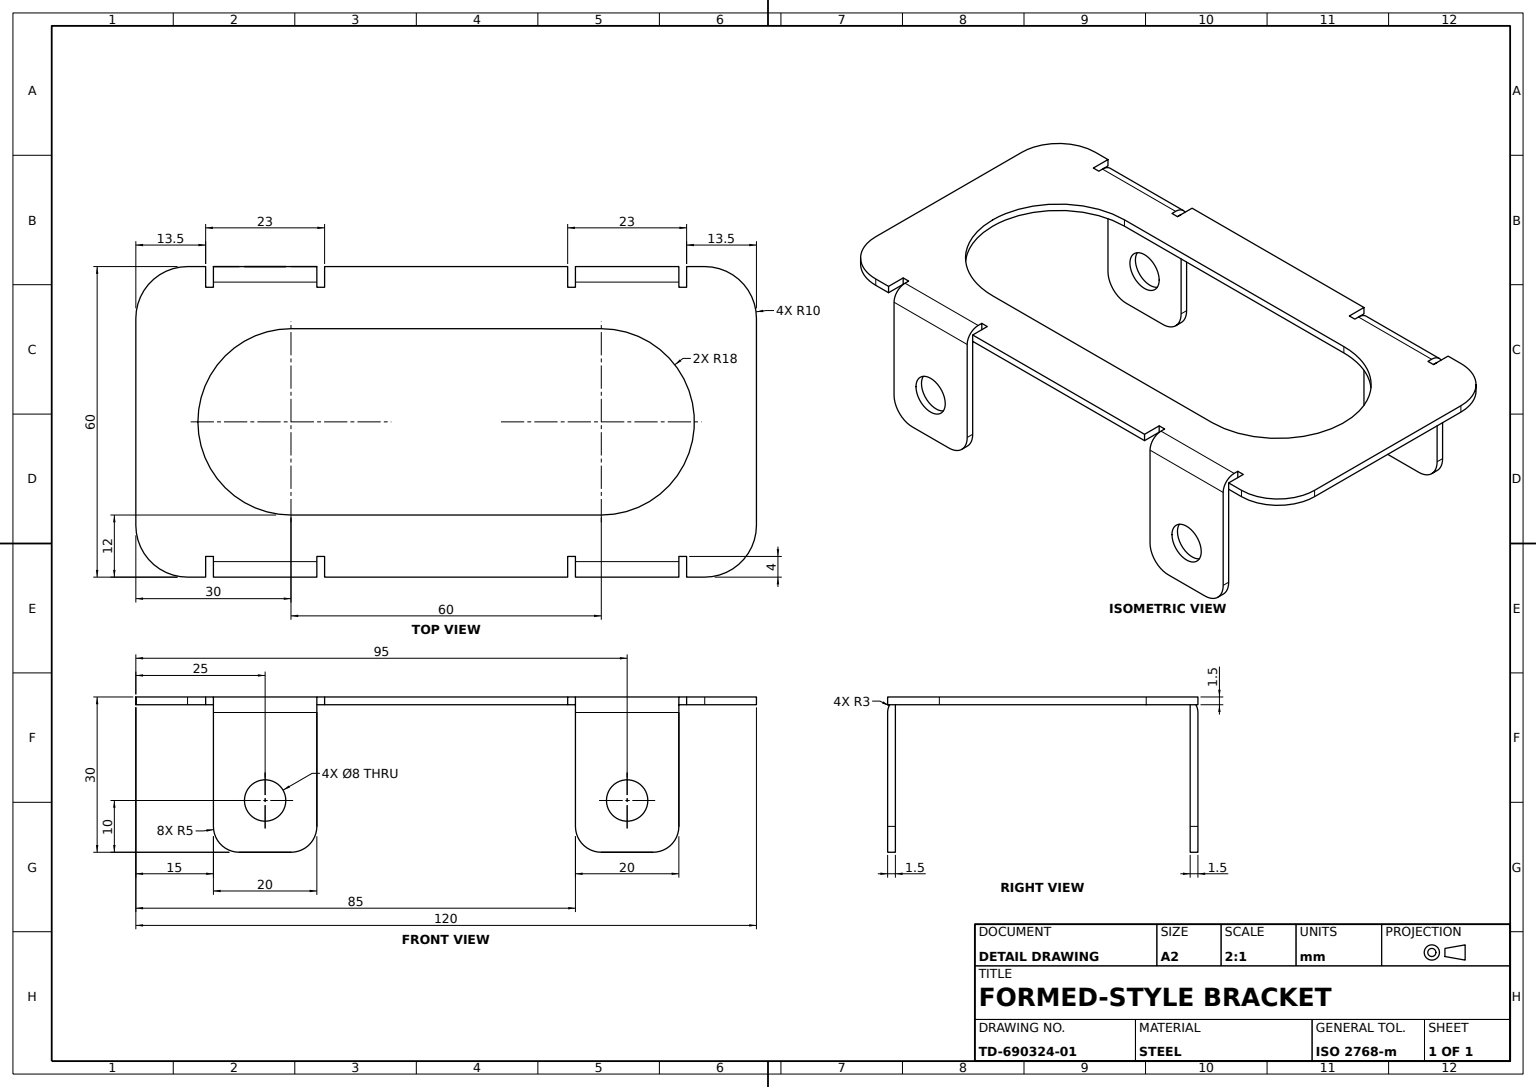
solid
v1 (-28.5,-18.5,39)
v2 (-28.5,-18.5,31)
e1 v1 v2 CIRCLE(AX(P(-28.5,-18.5,35),D(-1,0,0),D(0,0,1)),4)
e2 v2 v1 CIRCLE(AX(P(-28.5,-18.5,35),D(-1,0,0),D(0,0,1)),4)
v3 (-28.5,0,25)
v4 (-28.5,0,45)
e3 v3 v4 LINE
v5 (-28.5,-23.5,45)
e4 v5 v4 LINE
v6 (-28.5,-28.5,40)
e5 v6 v5 CIRCLE(AX(P(-28.5,-23.5,40),D(-1,0,0),D(0,0,1)),5)
v7 (-28.5,-28.5,30)
e6 v7 v6 LINE
v8 (-28.5,-23.5,25)
e7 v8 v7 CIRCLE(AX(P(-28.5,-23.5,30),D(-1,0,0),D(0,0,1)),5)
e8 v3 v8 LINE
face PLANE(AX(P(-28.5,-23.5,30),D(-1,0,0),D(0,0,1))) rev [e1 e2] [e3 -e4 -e5 -e6 -e7 -e8]
v9 (-30,-18.5,-39)
v10 (-30,-18.5,-31)
e9 v9 v10 CIRCLE(AX(P(-30,-18.5,-35),D(-1,0,0),D(0,0,1)),4)
e10 v10 v9 CIRCLE(AX(P(-30,-18.5,-35),D(-1,0,0),D(0,0,1)),4)
v11 (-30,-28.5,-40)
v12 (-30,-28.5,-30)
e11 v11 v12 LINE
v13 (-30,-23.5,-25)
e12 v12 v13 CIRCLE(AX(P(-30,-23.5,-30),D(-1,0,0),D(0,0,1)),5)
v14 (-30,-1.5,-25)
e13 v14 v13 LINE
v15 (-30,-1.5,-45)
e14 v14 v15 LINE
v16 (-30,-23.5,-45)
e15 v15 v16 LINE
e16 v16 v11 CIRCLE(AX(P(-30,-23.5,-40),D(-1,0,0),D(0,0,1)),5)
face PLANE(AX(P(-30,1.5,-45),D(1,0,0),D(0,0,-1))) rev [-e9 -e10] [e11 e12 -e13 e14 e15 e16]
v17 (-26,1.5,-46.5)
v18 (-26,1.5,-45)
e17 v17 v18 LINE
v19 (-26,0,-46.5)
e18 v17 v19 LINE
v20 (-26,0,-45)
e19 v19 v20 LINE
e20 v18 v20 LINE
face PLANE(AX(P(-26,1.5,-46.5),D(1,0,0),D(0,0,-1))) rev [-e17 e18 e19 -e20]
v21 (18,0,-30)
v22 (18,1.5,-30)
e21 v21 v22 LINE
v23 (-18,1.5,-30)
e22 v22 v23 CIRCLE(AX(P(0,1.5,-30),D(0,1,0),D(0,0,1)),18)
v24 (-18,0,-30)
e23 v24 v23 LINE
e24 v21 v24 CIRCLE(AX(P(0,0,-30),D(0,1,0),D(0,0,1)),18)
face CYL(AX(P(0,0,-30),D(0,1,0),D(0,0,1)),18) rev [e21 e22 -e23 -e24]
v25 (-18,1.5,30)
e25 v23 v25 LINE
v26 (-18,0,30)
e26 v26 v25 LINE
e27 v24 v26 LINE
face PLANE(AX(P(-18,0,30),D(-1,0,0),D(0,0,1))) rev [e23 e25 -e26 -e27]
v27 (27,1.5,-45)
v28 (30,-1.5,-45)
e28 v27 v28 CIRCLE(AX(P(27,-1.5,-45),D(0,0,-1),D(1,0,0)),3)
v29 (27,1.5,-25)
e29 v29 v27 LINE
v30 (30,-1.5,-25)
e30 v30 v29 CIRCLE(AX(P(27,-1.5,-25),D(0,0,1),D(-1,0,0)),3)
e31 v28 v30 LINE
face CYL(AX(P(27,-1.5,50),D(0,0,1),D(1,0,0)),3) [-e28 -e29 -e30 -e31]
v31 (26,0,-46.5)
v32 (30,0,-46.5)
e32 v31 v32 LINE
v33 (30,1.5,-46.5)
e33 v33 v32 LINE
v34 (26,1.5,-46.5)
e34 v34 v33 LINE
e35 v34 v31 LINE
face PLANE(AX(P(26,1.5,-46.5),D(0,0,-1),D(-1,0,0))) rev [e32 -e33 -e34 e35]
v35 (-26,0,45)
e36 v4 v35 LINE
v36 (-26,1.5,45)
e37 v36 v35 LINE
v37 (-27,1.5,45)
e38 v37 v36 LINE
v38 (-30,-1.5,45)
e39 v37 v38 CIRCLE(AX(P(-27,-1.5,45),D(0,0,1),D(-1,0,0)),3)
v39 (-30,-23.5,45)
e40 v38 v39 LINE
e41 v5 v39 LINE
face PLANE(AX(P(-30,1.5,45),D(0,0,-1),D(-1,0,0))) rev [e4 e36 -e37 -e38 e39 e40 -e41]
v40 (-28.5,-23.5,-25)
e42 v40 v13 LINE
v41 (-28.5,-28.5,-30)
e43 v41 v12 LINE
e44 v41 v40 CIRCLE(AX(P(-28.5,-23.5,-30),D(-1,0,0),D(0,0,1)),5)
face CYL(AX(P(-28.5,-23.5,-30),D(-1,0,0),D(0,0,1)),5) [e42 -e12 -e43 e44]
v42 (-30,1.5,-23.5)
v43 (-30,0,-23.5)
e45 v42 v43 LINE
v44 (-26,1.5,-23.5)
e46 v44 v42 LINE
v45 (-26,0,-23.5)
e47 v44 v45 LINE
e48 v45 v43 LINE
face PLANE(AX(P(-30,1.5,-23.5),D(0,0,1),D(1,0,0))) rev [-e45 -e46 e47 e48]
v46 (30,0,23.5)
v47 (30,0,-23.5)
e49 v46 v47 LINE
v48 (30,1.5,-23.5)
e50 v48 v47 LINE
v49 (30,1.5,23.5)
e51 v49 v48 LINE
e52 v49 v46 LINE
face PLANE(AX(P(30,1.5,-23.5),D(-1,0,0),D(0,0,1))) rev [e49 -e50 -e51 e52]
v50 (20,0,-60)
v51 (-20,0,-60)
e53 v50 v51 LINE
v52 (-20,1.5,-60)
e54 v52 v51 LINE
v53 (20,1.5,-60)
e55 v53 v52 LINE
e56 v53 v50 LINE
face PLANE(AX(P(-20,1.5,-60),D(0,0,1),D(1,0,0))) rev [e53 -e54 -e55 e56]
v54 (-28.5,-23.5,-45)
v55 (-28.5,-28.5,-40)
e57 v54 v55 CIRCLE(AX(P(-28.5,-23.5,-40),D(-1,0,0),D(0,0,1)),5)
e58 v55 v11 LINE
e59 v54 v16 LINE
face CYL(AX(P(-28.5,-23.5,-40),D(-1,0,0),D(0,0,1)),5) [e57 e58 -e16 -e59]
v56 (-30,-18.5,39)
e60 v1 v56 LINE
v57 (-30,-18.5,31)
e61 v56 v57 CIRCLE(AX(P(-30,-18.5,35),D(-1,0,0),D(0,0,1)),4)
e62 v2 v57 LINE
face CYL(AX(P(-28.5,-18.5,35),D(-1,0,0),D(0,0,1)),4) rev [e60 e61 -e62 -e1]
v58 (30,-18.5,39)
v59 (30,-18.5,31)
e63 v58 v59 CIRCLE(AX(P(30,-18.5,35),D(1,0,0),D(0,0,-1)),4)
e64 v59 v58 CIRCLE(AX(P(30,-18.5,35),D(1,0,0),D(0,0,-1)),4)
v60 (30,-28.5,30)
v61 (30,-23.5,25)
e65 v60 v61 CIRCLE(AX(P(30,-23.5,30),D(1,0,0),D(0,0,-1)),5)
v62 (30,-1.5,25)
e66 v62 v61 LINE
v63 (30,-1.5,45)
e67 v62 v63 LINE
v64 (30,-23.5,45)
e68 v63 v64 LINE
v65 (30,-28.5,40)
e69 v64 v65 CIRCLE(AX(P(30,-23.5,40),D(1,0,0),D(0,0,-1)),5)
e70 v65 v60 LINE
face PLANE(AX(P(30,1.5,25),D(-1,0,0),D(0,0,1))) rev [-e63 -e64] [e65 -e66 e67 e68 e69 e70]
v66 (28.5,-18.5,-31)
v67 (30,-18.5,-31)
e71 v66 v67 LINE
v68 (30,-18.5,-39)
e72 v67 v68 CIRCLE(AX(P(30,-18.5,-35),D(1,0,0),D(0,0,-1)),4)
v69 (28.5,-18.5,-39)
e73 v69 v68 LINE
e74 v66 v69 CIRCLE(AX(P(28.5,-18.5,-35),D(1,0,0),D(0,0,-1)),4)
face CYL(AX(P(28.5,-18.5,-35),D(1,0,0),D(0,0,-1)),4) rev [e71 e72 -e73 -e74]
e75 v55 v41 LINE
v70 (-28.5,0,-45)
e76 v70 v54 LINE
v71 (-28.5,0,-25)
e77 v70 v71 LINE
e78 v40 v71 LINE
v72 (-28.5,-18.5,-39)
v73 (-28.5,-18.5,-31)
e79 v72 v73 CIRCLE(AX(P(-28.5,-18.5,-35),D(-1,0,0),D(0,0,1)),4)
e80 v73 v72 CIRCLE(AX(P(-28.5,-18.5,-35),D(-1,0,0),D(0,0,1)),4)
face PLANE(AX(P(-28.5,-23.5,-40),D(-1,0,0),D(0,0,1))) rev [-e75 -e57 -e76 e77 -e78 -e44] [e79 e80]
v74 (26,1.5,-23.5)
v75 (26,1.5,-25)
e81 v74 v75 LINE
v76 (26,0,-23.5)
e82 v74 v76 LINE
v77 (26,0,-25)
e83 v76 v77 LINE
e84 v75 v77 LINE
face PLANE(AX(P(26,1.5,-25),D(-1,0,0),D(0,0,1))) rev [-e81 e82 e83 -e84]
v78 (30,-23.5,-25)
e85 v30 v78 LINE
v79 (30,-28.5,-30)
e86 v78 v79 CIRCLE(AX(P(30,-23.5,-30),D(1,0,0),D(0,0,-1)),5)
v80 (30,-28.5,-40)
e87 v79 v80 LINE
v81 (30,-23.5,-45)
e88 v80 v81 CIRCLE(AX(P(30,-23.5,-40),D(1,0,0),D(0,0,-1)),5)
e89 v28 v81 LINE
e90 v68 v67 CIRCLE(AX(P(30,-18.5,-35),D(1,0,0),D(0,0,-1)),4)
face PLANE(AX(P(30,1.5,-45),D(-1,0,0),D(0,0,1))) rev [e31 e85 e86 e87 e88 -e89] [-e90 -e72]
v82 (26,1.5,23.5)
v83 (26,0,23.5)
e91 v82 v83 LINE
e92 v83 v46 LINE
e93 v82 v49 LINE
face PLANE(AX(P(26,1.5,23.5),D(0,0,-1),D(-1,0,0))) rev [e91 e92 -e52 -e93]
v84 (27,1.5,45)
e94 v63 v84 CIRCLE(AX(P(27,-1.5,45),D(0,0,1),D(-1,0,0)),3)
v85 (26,1.5,45)
e95 v85 v84 LINE
v86 (26,0,45)
e96 v85 v86 LINE
v87 (28.5,0,45)
e97 v86 v87 LINE
v88 (28.5,-23.5,45)
e98 v87 v88 LINE
e99 v88 v64 LINE
face PLANE(AX(P(26,1.5,45),D(0,0,-1),D(-1,0,0))) rev [-e68 e94 -e95 e96 e97 e98 e99]
e100 v73 v10 LINE
e101 v72 v9 LINE
face CYL(AX(P(-28.5,-18.5,-35),D(-1,0,0),D(0,0,1)),4) rev [e100 e10 -e101 -e80]
v89 (30,1.5,50)
v90 (30,0,50)
e102 v89 v90 LINE
v91 (20,1.5,60)
e103 v91 v89 CIRCLE(AX(P(20,1.5,50),D(0,1,0),D(0,0,1)),10)
v92 (20,0,60)
e104 v91 v92 LINE
e105 v92 v90 CIRCLE(AX(P(20,0,50),D(0,1,0),D(0,0,1)),10)
face CYL(AX(P(20,1.5,50),D(0,-1,0),D(0,0,-1)),10) [-e102 -e103 e104 e105]
v93 (-30,1.5,-46.5)
v94 (-30,0,-46.5)
e106 v93 v94 LINE
v95 (-30,1.5,-50)
e107 v95 v93 LINE
v96 (-30,0,-50)
e108 v95 v96 LINE
e109 v96 v94 LINE
face PLANE(AX(P(-30,1.5,-50),D(1,0,0),D(0,0,-1))) rev [-e106 -e107 e108 e109]
v97 (28.5,-23.5,-25)
e110 v97 v78 LINE
v98 (28.5,-28.5,-30)
e111 v97 v98 CIRCLE(AX(P(28.5,-23.5,-30),D(1,0,0),D(0,0,-1)),5)
e112 v98 v79 LINE
face CYL(AX(P(28.5,-23.5,-30),D(1,0,0),D(0,0,-1)),5) [-e110 e111 e112 -e86]
v99 (-30,-23.5,25)
e113 v8 v99 LINE
v100 (-30,-1.5,25)
e114 v100 v99 LINE
v101 (-27,1.5,25)
e115 v100 v101 CIRCLE(AX(P(-27,-1.5,25),D(0,0,-1),D(1,0,0)),3)
v102 (-26,1.5,25)
e116 v102 v101 LINE
v103 (-26,0,25)
e117 v102 v103 LINE
e118 v103 v3 LINE
face PLANE(AX(P(-30,1.5,25),D(0,0,1),D(1,0,0))) rev [e8 e113 -e114 e115 -e116 e117 e118]
v104 (28.5,-28.5,40)
e119 v88 v104 CIRCLE(AX(P(28.5,-23.5,40),D(1,0,0),D(0,0,-1)),5)
e120 v104 v65 LINE
face CYL(AX(P(28.5,-23.5,40),D(1,0,0),D(0,0,-1)),5) [e119 e120 -e69 -e99]
v105 (26,1.5,46.5)
e121 v105 v85 LINE
v106 (26,0,46.5)
e122 v105 v106 LINE
e123 v106 v86 LINE
face PLANE(AX(P(26,1.5,45),D(-1,0,0),D(0,0,1))) rev [-e121 e122 e123 -e96]
v107 (26,1.5,25)
e124 v107 v82 LINE
v108 (26,0,25)
e125 v107 v108 LINE
e126 v108 v83 LINE
face PLANE(AX(P(26,1.5,23.5),D(-1,0,0),D(0,0,1))) rev [-e124 e125 e126 -e91]
v109 (28.5,-28.5,30)
e127 v104 v109 LINE
v110 (28.5,0,25)
e128 v87 v110 LINE
v111 (28.5,-23.5,25)
e129 v111 v110 LINE
e130 v109 v111 CIRCLE(AX(P(28.5,-23.5,30),D(1,0,0),D(0,0,-1)),5)
v112 (28.5,-18.5,39)
v113 (28.5,-18.5,31)
e131 v112 v113 CIRCLE(AX(P(28.5,-18.5,35),D(1,0,0),D(0,0,-1)),4)
e132 v113 v112 CIRCLE(AX(P(28.5,-18.5,35),D(1,0,0),D(0,0,-1)),4)
face PLANE(AX(P(28.5,-23.5,40),D(1,0,0),D(0,0,-1))) rev [-e127 -e119 -e98 e128 -e129 -e130] [e131 e132]
v114 (-27,1.5,-45)
v115 (-27,1.5,-25)
e133 v114 v115 LINE
e134 v15 v114 CIRCLE(AX(P(-27,-1.5,-45),D(0,0,-1),D(1,0,0)),3)
e135 v115 v14 CIRCLE(AX(P(-27,-1.5,-25),D(0,0,1),D(-1,0,0)),3)
face CYL(AX(P(-27,-1.5,50),D(0,0,-1),D(-1,0,0)),3) [-e133 -e134 -e14 -e135]
v116 (30,1.5,-50)
e136 v33 v116 LINE
e137 v116 v53 CIRCLE(AX(P(20,1.5,-50),D(0,1,0),D(0,0,-1)),10)
e138 v52 v95 CIRCLE(AX(P(-20,1.5,-50),D(0,1,0),D(0,0,1)),10)
e139 v93 v17 LINE
e140 v18 v114 LINE
v117 (-26,1.5,-25)
e141 v115 v117 LINE
e142 v117 v44 LINE
v118 (-30,1.5,23.5)
e143 v42 v118 LINE
v119 (-26,1.5,23.5)
e144 v118 v119 LINE
e145 v119 v102 LINE
e146 v101 v37 LINE
v120 (-26,1.5,46.5)
e147 v36 v120 LINE
v121 (-30,1.5,46.5)
e148 v120 v121 LINE
v122 (-30,1.5,50)
e149 v121 v122 LINE
v123 (-20,1.5,60)
e150 v122 v123 CIRCLE(AX(P(-20,1.5,50),D(0,1,0),D(0,0,1)),10)
e151 v123 v91 LINE
v124 (30,1.5,46.5)
e152 v89 v124 LINE
e153 v124 v105 LINE
v125 (27,1.5,25)
e154 v84 v125 LINE
e155 v125 v107 LINE
e156 v48 v74 LINE
e157 v75 v29 LINE
v126 (26,1.5,-45)
e158 v27 v126 LINE
e159 v126 v34 LINE
v127 (0,1.5,48)
e160 v25 v127 CIRCLE(AX(P(0,1.5,30),D(0,1,0),D(0,0,1)),18)
v128 (18,1.5,30)
e161 v128 v22 LINE
e162 v127 v128 CIRCLE(AX(P(0,1.5,30),D(0,1,0),D(0,0,1)),18)
face PLANE(AX(P(-20,1.5,50),D(0,1,0),D(0,0,1))) [e136 e137 e55 e138 e107 e139 e17 e140 e133 e141 e142 e46 e143 e144 e145 e116 e146 e38 e147 e148 e149 e150 e151 e103 e152 e153 e121 e95 e154 e155 e124 e93 e51 e156 e81 e157 e29 e158 e159 e34] [-e160 -e25 -e22 -e161 -e162]
v129 (-30,0,23.5)
e163 v43 v129 LINE
e164 v118 v129 LINE
face PLANE(AX(P(-30,1.5,-23.5),D(1,0,0),D(0,0,-1))) rev [e163 -e164 -e143 e45]
v130 (30,0,46.5)
e165 v130 v106 LINE
e166 v124 v130 LINE
face PLANE(AX(P(26,1.5,46.5),D(0,0,1),D(1,0,0))) rev [e165 -e122 -e153 e166]
v131 (-30,0,46.5)
e167 v121 v131 LINE
v132 (-30,0,50)
e168 v131 v132 LINE
e169 v122 v132 LINE
face PLANE(AX(P(-30,1.5,46.5),D(1,0,0),D(0,0,-1))) rev [e167 e168 -e169 -e149]
v133 (-30,-28.5,30)
e170 v99 v133 CIRCLE(AX(P(-30,-23.5,30),D(-1,0,0),D(0,0,1)),5)
e171 v7 v133 LINE
face CYL(AX(P(-28.5,-23.5,30),D(-1,0,0),D(0,0,1)),5) [-e170 -e113 e7 e171]
v134 (0,0,48)
e172 v26 v134 CIRCLE(AX(P(0,0,30),D(0,1,0),D(0,0,1)),18)
e173 v134 v127 LINE
face CYL(AX(P(0,0,30),D(0,1,0),D(0,0,1)),18) rev [-e172 e26 e160 -e173]
v135 (-30,-28.5,40)
e174 v135 v39 CIRCLE(AX(P(-30,-23.5,40),D(-1,0,0),D(0,0,1)),5)
e175 v6 v135 LINE
face CYL(AX(P(-28.5,-23.5,40),D(-1,0,0),D(0,0,1)),5) [e5 e41 -e174 -e175]
v136 (-26,0,-25)
e176 v71 v136 LINE
e177 v117 v136 LINE
face PLANE(AX(P(-30,1.5,-25),D(0,0,-1),D(-1,0,0))) rev [e176 -e177 -e141 e135 e13 -e42 e78]
e178 v109 v60 LINE
e179 v111 v61 LINE
face CYL(AX(P(28.5,-23.5,30),D(1,0,0),D(0,0,-1)),5) [-e65 -e178 e130 e179]
e180 v110 v108 LINE
e181 v125 v62 CIRCLE(AX(P(27,-1.5,25),D(0,0,-1),D(1,0,0)),3)
face PLANE(AX(P(26,1.5,25),D(0,0,1),D(1,0,0))) rev [-e179 e129 e180 -e125 -e155 e181 e66]
v137 (18,0,30)
e182 v137 v128 LINE
e183 v134 v137 CIRCLE(AX(P(0,0,30),D(0,1,0),D(0,0,1)),18)
face CYL(AX(P(0,0,30),D(0,1,0),D(0,0,1)),18) rev [e173 e162 -e182 -e183]
e184 v20 v70 LINE
face PLANE(AX(P(-30,1.5,-45),D(0,0,1),D(1,0,0))) rev [e20 e184 e76 e59 -e15 e134 -e140]
face PLANE(AX(P(-28.5,-28.5,-40),D(0,-1,0),D(0,0,-1))) [-e58 e75 e43 -e11]
v138 (-26,0,23.5)
e185 v119 v138 LINE
e186 v129 v138 LINE
face PLANE(AX(P(-30,1.5,23.5),D(0,0,-1),D(-1,0,0))) rev [-e185 -e144 e164 e186]
e187 v38 v100 LINE
e188 v133 v135 LINE
e189 v57 v56 CIRCLE(AX(P(-30,-18.5,35),D(-1,0,0),D(0,0,1)),4)
face PLANE(AX(P(-30,1.5,25),D(1,0,0),D(0,0,-1))) rev [-e40 e187 e114 e170 e188 e174] [-e189 -e61]
v139 (26,0,-45)
e190 v126 v139 LINE
v140 (28.5,-23.5,-45)
e191 v140 v81 LINE
v141 (28.5,0,-45)
e192 v140 v141 LINE
e193 v141 v139 LINE
face PLANE(AX(P(26,1.5,-45),D(0,0,1),D(1,0,0))) rev [-e190 -e158 e28 e89 -e191 e192 e193]
face CYL(AX(P(-27,-1.5,50),D(0,0,-1),D(-1,0,0)),3) [-e187 -e39 -e146 -e115]
v142 (30,0,-50)
e194 v116 v142 LINE
e195 v142 v50 CIRCLE(AX(P(20,0,-50),D(0,1,0),D(0,0,-1)),10)
face CYL(AX(P(20,1.5,-50),D(0,-1,0),D(0,0,-1)),10) [e194 e195 -e56 -e137]
v143 (28.5,-28.5,-40)
e196 v143 v140 CIRCLE(AX(P(28.5,-23.5,-40),D(1,0,0),D(0,0,-1)),5)
e197 v143 v80 LINE
face CYL(AX(P(28.5,-23.5,-40),D(1,0,0),D(0,0,-1)),5) [e196 e191 -e88 -e197]
face PLANE(AX(P(28.5,-28.5,40),D(0,-1,0),D(0,0,-1))) [-e120 e127 e178 -e70]
face CYL(AX(P(27,-1.5,50),D(0,0,1),D(1,0,0)),3) [-e67 -e181 -e154 -e94]
e198 v32 v142 LINE
face PLANE(AX(P(30,1.5,-50),D(-1,0,0),D(0,0,1))) rev [-e136 e33 e198 -e194]
e199 v136 v45 LINE
face PLANE(AX(P(-26,1.5,-25),D(1,0,0),D(0,0,-1))) rev [-e47 -e142 e177 e199]
e200 v94 v19 LINE
face PLANE(AX(P(-30,1.5,-46.5),D(0,0,-1),D(-1,0,0))) rev [e200 -e18 -e139 e106]
face PLANE(AX(P(-28.5,-28.5,30),D(0,-1,0),D(0,0,-1))) [e6 e175 -e188 -e171]
e201 v47 v76 LINE
face PLANE(AX(P(26,1.5,-23.5),D(0,0,1),D(1,0,0))) rev [-e82 -e156 e50 e201]
e202 v69 v66 CIRCLE(AX(P(28.5,-18.5,-35),D(1,0,0),D(0,0,-1)),4)
face CYL(AX(P(28.5,-18.5,-35),D(1,0,0),D(0,0,-1)),4) rev [-e202 e73 e90 -e71]
e203 v138 v103 LINE
face PLANE(AX(P(-26,1.5,23.5),D(1,0,0),D(0,0,-1))) rev [-e117 -e145 e185 e203]
v144 (-20,0,60)
e204 v123 v144 LINE
e205 v144 v92 LINE
face PLANE(AX(P(-20,1.5,60),D(0,0,-1),D(-1,0,0))) rev [-e104 -e151 e204 e205]
e206 v139 v31 LINE
face PLANE(AX(P(26,1.5,-46.5),D(-1,0,0),D(0,0,1))) rev [-e159 e190 e206 -e35]
e207 v113 v59 LINE
e208 v112 v58 LINE
face CYL(AX(P(28.5,-18.5,35),D(1,0,0),D(0,0,-1)),4) rev [e207 e64 -e208 -e132]
e209 v90 v130 LINE
face PLANE(AX(P(30,1.5,46.5),D(-1,0,0),D(0,0,1))) rev [e209 -e166 -e152 e102]
v145 (28.5,0,-25)
e210 v77 v145 LINE
e211 v145 v97 LINE
face PLANE(AX(P(26,1.5,-25),D(0,0,-1),D(-1,0,0))) rev [-e85 e30 -e157 e84 e210 e211 e110]
face CYL(AX(P(-28.5,-18.5,35),D(-1,0,0),D(0,0,1)),4) rev [e189 -e60 -e2 e62]
e212 v132 v144 CIRCLE(AX(P(-20,0,50),D(0,1,0),D(0,0,1)),10)
face CYL(AX(P(-20,1.5,50),D(0,-1,0),D(0,0,-1)),10) [e212 -e204 -e150 e169]
face CYL(AX(P(-28.5,-18.5,-35),D(-1,0,0),D(0,0,1)),4) rev [-e100 -e79 e101 e9]
e213 v137 v21 LINE
face PLANE(AX(P(18,0,30),D(1,0,0),D(0,0,-1))) rev [e161 -e21 -e213 e182]
v146 (-26,0,46.5)
e214 v35 v146 LINE
e215 v120 v146 LINE
face PLANE(AX(P(-26,1.5,45),D(1,0,0),D(0,0,-1))) rev [e37 e214 -e215 -e147]
e216 v145 v141 LINE
e217 v98 v143 LINE
face PLANE(AX(P(28.5,-23.5,-30),D(1,0,0),D(0,0,-1))) rev [e74 e202] [-e111 -e211 e216 -e192 -e196 -e217]
e218 v51 v96 CIRCLE(AX(P(-20,0,-50),D(0,1,0),D(0,0,1)),10)
e219 v146 v131 LINE
face PLANE(AX(P(-20,0,50),D(0,1,0),D(0,0,1))) rev [-e218 -e53 -e195 -e198 -e32 -e206 -e193 -e216 -e210 -e83 -e201 -e49 -e92 -e126 -e180 -e128 -e97 -e123 -e165 -e209 -e105 -e205 -e212 -e168 -e219 -e214 -e36 -e3 -e118 -e203 -e186 -e163 -e48 -e199 -e176 -e77 -e184 -e19 -e200 -e109] [e183 e213 e24 e27 e172]
face CYL(AX(P(-20,1.5,-50),D(0,-1,0),D(0,0,-1)),10) [-e138 e54 e218 -e108]
face PLANE(AX(P(-30,1.5,46.5),D(0,0,1),D(1,0,0))) rev [-e167 -e148 e215 e219]
face CYL(AX(P(28.5,-18.5,35),D(1,0,0),D(0,0,-1)),4) rev [-e207 -e131 e208 e63]
face PLANE(AX(P(28.5,-28.5,-30),D(0,-1,0),D(0,0,-1))) [-e87 -e112 e217 e197]
